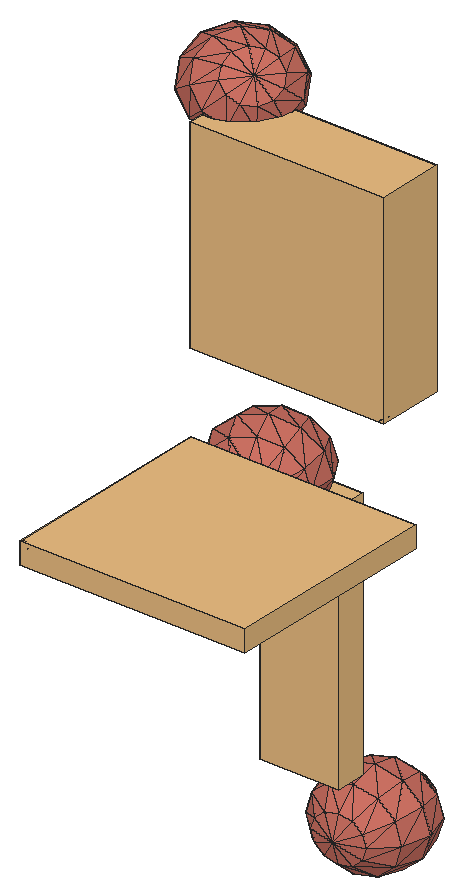
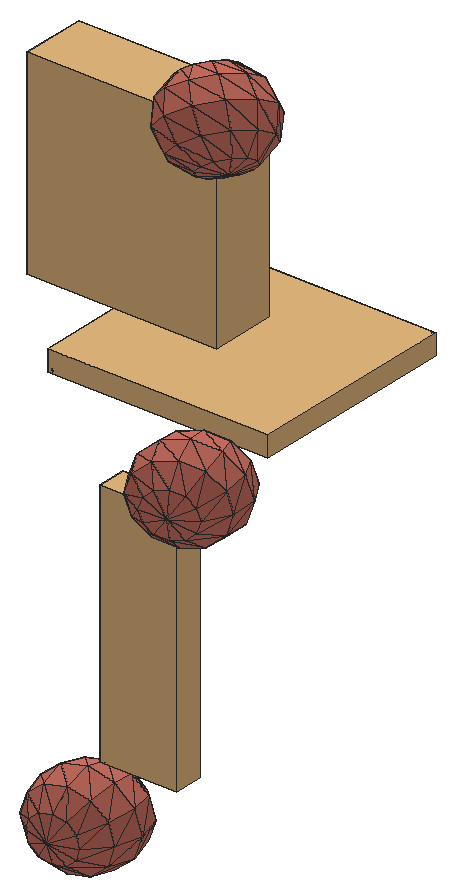
# SketchUp Ruby script. Lengths in inches.
U = 1.inch
M = Sketchup.active_model
def pt(a) = Geom::Point3d.new(a.map { |v| v * U })
def face(e, loops, mat)
  f = e.add_face(loops[0].map { |a| pt(a) })
  loops[1..].each { |l| e.add_face(l.map { |a| pt(a) }).erase! }
  f.material = f.back_material = mat if mat
  f
end
# faces: each face lists its corners as indices into pts; further lists are holes
def faces(e, pts, list, mat = nil) = list.each { |f| face(e, (f[0].is_a?(Array) ? f : [f]).map { |l| l.map { |i| pts[i] } }, mat) }
# xy, xz, yz: faces in a plane at the given z, y or x. An outline is a flat list of corners, or four numbers for a rectangle; further outlines are holes
def ring(l) = l.size == 4 ? [[l[0], l[1]], [l[2], l[1]], [l[2], l[3]], [l[0], l[3]]] : l.each_slice(2).to_a
def flat(e, list, mat, &to3) = list.each { |f| face(e, (f[0].is_a?(Array) ? f : [f]).map { |l| ring(l).map { |u, v| to3.(u, v) } }, mat) }
def xy(e, z, list, mat = nil) = flat(e, list, mat) { |x, y| [x, y, z] }
def xz(e, y, list, mat = nil) = flat(e, list, mat) { |x, z| [x, y, z] }
def yz(e, x, list, mat = nil) = flat(e, list, mat) { |y, z| [x, y, z] }
def lines(e, pts, list) = list.each { |a, b| e.add_line(pt(pts[a]), pt(pts[b])) }
# prism: a flat outline (further loops are holes) pulled along v
def prism(e, loops, v, mat = nil)
  f = face(e, loops, mat); d = Geom::Vector3d.new(v.map { |x| x * U })
  f.pushpull(f.normal.samedirection?(d) ? d.length : -d.length)
end
def box(e, o, s, mat = nil) = prism(e, [[o, [o[0] + s[0], o[1], o[2]], [o[0] + s[0], o[1] + s[1], o[2]], [o[0], o[1] + s[1], o[2]]]], [0, 0, s[2]], mat)
def at(x, y, z, deg = 0) = Geom::Transformation.translation(pt([x, y, z])) * Geom::Transformation.rotation(ORIGIN, Z_AXIS, deg.degrees)
def axes(o, x, y, z) = Geom::Transformation.new([*x, 0, *y, 0, *z, 0, *pt(o).to_a, 1])
def part(name) = M.definitions.add(name)
# library, detail: a bought-in or finely detailed component or shape, given as its bounding box
def library(name, o, s) = part(name).tap { |d| box(d.entities, o, s) }
def detail(e, o, s) = box(e.add_group.entities, o, s)
def put(e, d, t, mat = nil) = e.add_instance(d, t).tap { |i| i.material = mat if mat }
def group(e, t, mat = nil) = e.add_group.tap { |g| g.transformation = t; g.material = mat if mat }.entities
root = M.entities
M.materials.add("green").color = [174, 139, 102]
M.materials.add("vio").color = [206, 114, 100]
c1 = part("3DGeom~243_Defintion")
p = [[-200.91,-81.6,-448.49],[84.65,14.19,-493.26],[-94.16,-142.9,-462.11],[213.68,-130.85,-425.83],[389.77,0,-314.38],[-100.26,120.37,-469.67],
  [240.77,167.48,-392.24],[389.77,0,-314.38],[-311.32,-59.16,-385.97],[-291.49,159.24,-361.38],[27.26,290.09,-365],[-19.66,-226.64,-423.18],
  [-247.73,-261.7,-307.14],[-247.73,-261.7,-307.14],[-247.73,-261.7,-307.14],[252.27,-275.9,-285.45],[213.68,-130.85,-425.83],[434.32,-167.48,-152.28],
  [252.27,-275.9,-285.45],[213.68,-130.85,-425.83],[389.77,0,-314.38],[2.62,-310.38,-342.13],[-247.73,-261.7,-307.14],[252.27,-275.9,-285.45],
  [2.62,-310.38,-342.13],[240.77,167.48,-392.24],[461.41,130.85,-118.6875],[240.77,167.48,-392.24],[332.38,275.9,-186.12],[332.38,275.9,-186.12],
  [-395.79,-81.6,-291.3],[-247.73,-261.7,-307.14],[-395.79,-81.6,-291.3],[-291.49,159.24,-361.38],[-311.32,-59.16,-385.97],[-193.55,334.96,-239.96],
  [147.48,382.07,-162.53],[332.38,275.9,-186.12],[-193.55,334.96,-239.96],[147.48,382.07,-162.53],[27.26,290.09,-365],[-395.79,-81.6,-291.3],
  [-437.8,120.37,-197.41],[-291.49,159.24,-361.38],[-193.55,334.96,-239.96],[-291.49,159.24,-361.38],[2.62,-310.38,-342.13],[190.07,-382.08,-109.73],
  [-33.29,-371.6875,-240.68],[252.27,-275.9,-285.45],[-247.73,-261.7,-307.14],[500,-14.19,21.69],[-117.77,-394.125,-146.01],[-228.17,-371.6875,-83.49],
  [-334.93,-310.38,-69.87],[-334.93,-310.38,-69.87],[-409.43,-226.64,-108.8],[-247.73,-261.7,-307.14],[-431.7,-142.9,-189.85],[-395.79,-81.6,-291.3],
  [-247.73,-261.7,-307.14],[-247.73,-261.7,-307.14],[-395.79,-81.6,-291.3],[252.27,-275.9,-285.45],[362.5,-290.09,50.625],[190.07,-382.08,-109.73],
  [252.27,-275.9,-285.45],[362.5,-290.09,50.625],[43.75,-420.9375,54.25],[-362.5,290.09,-50.625],[-193.55,334.96,-239.96],[-362.5,290.09,-50.625],
  [-43.75,420.9375,-54.25],[-193.55,334.96,-239.96],[-193.55,334.96,-239.96],[147.48,382.07,-162.53],[-500,14.19,-21.69],[409.43,226.64,108.8],
  [334.93,310.39,69.87],[147.48,382.07,-162.53],[334.93,310.39,69.87],[332.38,275.9,-186.12],[147.48,382.07,-162.53],[228.17,371.6875,83.49],
  [334.93,310.39,69.87],[147.48,382.07,-162.53],[437.8,-120.37,197.41],[362.5,-290.09,50.625],[-147.48,-382.08,162.53],[431.7,142.9,189.85],
  [193.55,-334.97,239.96],[362.5,-290.09,50.625],[-461.41,-130.85,118.6875],[-332.38,-275.9,186.12],[-332.38,-275.9,186.12],[-334.93,-310.38,-69.87],
  [-332.38,-275.9,186.12],[-362.5,290.09,-50.625],[-190.07,382.08,109.73],[117.77,394.125,146.01],[-434.32,167.48,152.28],[-190.07,382.08,109.73],
  [395.79,81.6,291.3],[362.5,-290.09,50.625],[291.49,-159.24,361.38],[193.55,-334.97,239.96],[362.5,-290.09,50.625],[-27.26,-290.09,365],
  [-27.26,-290.09,365],[247.73,261.7,307.14],[334.93,310.39,69.87],[247.73,261.7,307.14],[247.73,261.7,307.14],[247.73,261.7,307.14],
  [-252.27,275.9,285.45],[-190.07,382.08,109.73],[-252.27,275.9,285.45],[33.29,371.6875,240.68],[-389.77,0,314.38],[247.73,261.7,307.14],
  [-147.48,-382.08,162.53],[-240.77,-167.48,392.24],[-332.38,-275.9,186.12],[-147.48,-382.08,162.53],[-27.26,-290.09,365],[-240.77,-167.48,392.24],
  [-240.77,-167.48,392.24],[247.73,261.7,307.14],[311.32,59.16,385.97],[193.55,-334.97,239.96],[100.26,-120.37,469.67],[193.55,-334.97,239.96],
  [291.49,-159.24,361.38],[-2.62,310.39,342.13],[247.73,261.7,307.14],[-252.27,275.9,285.45],[-213.68,130.85,425.83],[-213.68,130.85,425.83],
  [-2.62,310.39,342.13],[-252.27,275.9,285.45],[311.32,59.16,385.97],[395.79,81.6,291.3],[247.73,261.7,307.14],[200.91,81.6,448.49],
  [311.32,59.16,385.97],[94.16,142.9,462.11],[19.66,226.64,423.18],[-2.62,310.39,342.13],[-240.77,-167.48,392.24],[-213.68,130.85,425.83],
  [-389.77,0,314.38],[-213.68,130.85,425.83],[-2.62,310.39,342.13],[291.49,-159.24,361.38],[291.49,-159.24,361.38],[311.32,59.16,385.97],
  [-84.65,-14.19,493.26],[-240.77,-167.48,392.24],[-240.77,-167.48,392.24],[-213.68,130.85,425.83],[-213.68,130.85,425.83]]
faces(c1.entities,p,[[0,1,2],[2,1,3],[1,4,3],[0,5,1],[1,6,7],[5,6,1],[8,5,0],[8,9,5],
  [9,10,5],[5,10,6],[2,11,12],[0,2,13],[2,3,11],[8,0,14],[11,3,15],[16,17,18],
  [19,20,17],[11,21,22],[11,23,24],[25,26,20],[27,28,26],[10,29,6],[30,8,31],[32,33,34],
  [9,35,10],[10,36,37],[38,39,40],[41,42,43],[42,44,45],[46,47,48],[46,49,47],[46,48,50],
  [20,51,17],[20,26,51],[48,52,50],[52,53,50],[53,54,50],[55,56,57],[58,59,60],[56,58,61],
  [58,42,62],[63,64,65],[66,17,67],[48,68,52],[48,47,68],[42,69,70],[71,72,73],[74,72,75],
  [58,76,42],[76,69,42],[56,76,58],[28,77,26],[28,78,77],[79,80,81],[82,83,84],[72,83,85],
  [17,86,87],[17,51,86],[52,68,88],[52,88,53],[26,89,51],[26,77,89],[47,90,68],[47,91,90],
  [55,92,56],[56,92,76],[53,88,93],[53,94,95],[55,96,92],[97,98,72],[72,99,83],[98,99,72],
  [76,100,69],[100,101,69],[92,100,76],[51,102,86],[51,89,102],[103,104,105],[106,86,104],[68,107,88],
  [68,90,108],[77,78,109],[110,83,111],[83,99,112],[89,77,113],[100,114,115],[116,117,98],[98,117,99],
  [96,118,92],[92,118,100],[99,117,119],[118,114,100],[120,121,122],[123,124,125],[96,126,118],[102,89,127],
  [86,128,104],[86,102,128],[129,130,124],[131,132,130],[117,133,134],[135,133,117],[118,136,114],[137,138,139],
  [140,141,142],[143,144,142],[145,143,142],[146,145,142],[147,146,142],[148,149,150],[151,146,152],[153,143,130],
  [154,155,143],[124,156,157],[124,130,156],[158,156,159],[156,146,160],[156,145,146],[130,143,145],[130,145,156]],"vio")
c2 = part("3DGeom~210_Defintion")
p = [[-113.26,0,-500],[131.5625,-217.6,-424.04],[-130.88,-188.44,-443.1875],[151.92,0,-489.64],[-348.08,0,-376.38],[-358.26,108.8,-343.58],
  [-130.88,188.44,-443.1875],[-358.26,108.8,-343.58],[-348.08,0,-376.38],[358.76,-188.44,-291.27],[376.38,0,-348.08],[358.76,-188.44,-291.27],
  [131.5625,217.6,-424.04],[75.96,-376.89,-244.82],[-179.04,-326.4,-287.98],[75.96,-376.89,-244.82],[-358.26,-108.8,-343.58],[-179.04,-326.4,-287.98],
  [-348.08,0,-376.38],[-358.26,-108.8,-343.58],[-386.0625,188.44,-253.97],[-358.26,108.8,-343.58],[-386.0625,188.44,-253.97],[-179.04,326.4,-287.98],
  [131.5625,-217.6,-424.04],[310.6,-326.4,-136.0625],[75.96,-376.89,-244.82],[131.5625,-217.6,-424.04],[358.76,-188.44,-291.27],[358.76,188.44,-291.27],
  [75.96,376.89,-244.82],[358.76,188.44,-291.27],[131.5625,217.6,-424.04],[75.96,376.89,-244.82],[-348.08,0,-376.38],[-358.26,-108.8,-343.58],
  [-489.64,0,-151.92],[-358.26,108.8,-343.58],[376.38,0,-348.08],[489.82,-108.8,-80.46],[358.76,-188.44,-291.27],[376.38,0,-348.08],
  [500,0,-113.26],[358.76,188.44,-291.27],[376.38,0,-348.08],[-358.26,-108.8,-343.58],[-179.04,-326.4,-287.98],[-386.0625,-188.44,-253.97],
  [-386.0625,-188.44,-253.97],[-386.0625,188.44,-253.97],[358.76,-188.44,-291.27],[462.02,-188.44,9.15],[310.6,-326.4,-136.0625],[358.76,-188.44,-291.27],
  [358.76,188.44,-291.27],[489.82,108.8,-80.46],[310.6,326.4,-136.0625],[358.76,188.44,-291.27],[75.96,376.89,-244.82],[310.6,326.4,-136.0625],
  [358.76,188.44,-291.27],[-179.04,-326.4,-287.98],[0,-435.19,0],[-244.82,-376.89,-75.96],[-179.04,-326.4,-287.98],[-179.04,-326.4,-287.98],
  [-244.82,-376.89,-75.96],[-424.04,217.6,-131.5625],[-179.04,326.4,-287.98],[-244.82,376.89,-75.96],[-179.04,326.4,-287.98],[-244.82,376.89,-75.96],
  [75.96,376.89,-244.82],[-179.04,326.4,-287.98],[-424.04,-217.6,-131.5625],[244.82,-376.89,75.96],[0,435.19,0],[75.96,376.89,-244.82],
  [-244.82,376.89,-75.96],[75.96,376.89,-244.82],[-462.02,-188.44,-9.15],[-489.82,-108.8,80.46],[-500,0,113.26],[-489.82,108.8,80.46],
  [-462.02,188.44,-9.15],[310.6,-326.4,-136.0625],[424.04,-217.6,131.5625],[244.82,-376.89,75.96],[310.6,-326.4,-136.0625],[310.6,326.4,-136.0625],
  [462.02,188.44,9.15],[244.82,376.89,75.96],[310.6,326.4,-136.0625],[244.82,376.89,75.96],[-310.6,-326.4,136.0625],[489.64,0,151.92],
  [-244.82,-376.89,-75.96],[-75.96,-376.89,244.82],[-244.82,-376.89,-75.96],[-310.6,-326.4,136.0625],[-310.6,326.4,136.0625],[-310.6,326.4,136.0625],
  [-244.82,376.89,-75.96],[-358.76,-188.44,291.27],[179.04,-326.39,287.98],[179.04,-326.39,287.98],[-310.6,326.4,136.0625],[-75.96,376.89,244.82],
  [424.04,217.6,131.5625],[244.82,376.89,75.96],[244.82,-376.89,75.96],[386.0625,-188.44,253.97],[179.04,-326.39,287.98],[244.82,-376.89,75.96],
  [386.0625,-188.44,253.97],[179.04,326.4,287.98],[244.82,376.89,75.96],[179.04,326.4,287.98],[-376.38,0,348.08],[-358.76,188.44,291.27],
  [386.0625,-188.44,253.97],[386.0625,188.44,253.97],[179.04,326.4,287.98],[-310.6,-326.4,136.0625],[-131.5625,-217.6,424.04],[-310.6,-326.4,136.0625],
  [-131.5625,-217.6,424.04],[-358.76,-188.44,291.27],[-358.76,188.44,291.27],[-310.6,326.4,136.0625],[358.26,-108.8,343.58],[386.0625,-188.44,253.97],
  [348.08,0,376.38],[358.26,-108.8,343.58],[358.26,108.8,343.58],[348.08,0,376.38],[358.26,108.8,343.58],[-75.96,-376.89,244.82],
  [130.88,-188.44,443.1875],[-131.5625,-217.6,424.04],[-75.96,-376.89,244.82],[179.04,-326.39,287.98],[-358.76,188.44,291.27],[-131.5625,217.6,424.04],
  [-131.5625,217.6,424.04],[179.04,326.4,287.98],[-75.96,376.89,244.82],[386.0625,-188.44,253.97],[358.26,-108.8,343.58],[130.88,188.44,443.1875],
  [358.26,108.8,343.58],[386.0625,188.44,253.97],[386.0625,188.44,253.97],[179.04,326.4,287.98],[-131.5625,217.6,424.04],[179.04,326.4,287.98],
  [-358.76,-188.44,291.27],[-151.92,0,489.64],[-358.76,-188.44,291.27],[-376.38,0,348.08],[-376.38,0,348.08],[-131.5625,217.6,424.04],
  [-358.76,188.44,291.27],[348.08,0,376.38],[113.26,0,500],[-376.38,0,348.08],[-131.5625,217.6,424.04],[-131.5625,217.6,424.04]]
faces(c2.entities,p,[[0,1,2],[0,3,1],[4,0,2],[5,6,0],[7,0,8],[6,3,0],[3,9,1],[3,10,11],
  [6,12,3],[12,10,3],[2,13,14],[2,1,15],[16,2,17],[18,2,19],[20,6,21],[22,23,6],
  [23,12,6],[24,25,26],[27,28,25],[12,29,10],[30,31,32],[23,33,12],[34,35,36],[37,34,36],
  [38,39,40],[41,42,39],[43,42,44],[45,46,47],[35,48,36],[49,37,36],[50,51,52],[53,39,51],
  [54,55,42],[56,55,57],[58,59,60],[61,62,63],[64,26,62],[48,65,66],[67,68,49],[67,69,70],
  [71,72,73],[48,66,74],[48,74,36],[67,49,36],[26,75,62],[26,25,75],[76,59,77],[78,76,79],
  [74,80,36],[80,81,36],[81,82,36],[82,83,36],[83,84,36],[84,67,36],[85,86,87],[88,51,86],
  [89,90,55],[91,90,92],[76,93,59],[74,66,94],[74,94,80],[84,69,67],[39,42,95],[42,55,95],
  [51,39,95],[55,90,95],[96,62,97],[98,97,99],[84,100,69],[101,76,102],[80,94,103],[80,103,81],
  [83,100,84],[62,104,97],[62,75,105],[106,107,76],[107,93,76],[86,51,95],[90,108,95],[109,108,90],
  [110,111,112],[113,86,114],[115,108,116],[107,117,93],[81,103,118],[81,118,82],[82,119,83],[83,119,100],
  [82,118,119],[120,86,95],[108,121,95],[122,121,108],[123,97,124],[125,126,127],[128,107,129],[130,131,95],
  [132,133,95],[134,135,95],[121,136,95],[137,138,139],[140,141,138],[142,143,107],[144,145,146],[141,147,148],
  [149,150,151],[149,152,153],[141,148,138],[154,149,155],[156,139,157],[158,157,159],[160,161,162],[138,148,163],
  [164,163,150],[164,150,149],[165,157,166],[138,163,164],[139,164,157],[139,138,164],[157,149,167],[157,164,149]],"vio")
c3 = library("3DGeom~78_Defintion",[-59.29,-500,-155.55],[118.58,1000,311.1])
c4 = part("3DGeom~79_Defintion")
p = [[38.96,500,-125.75],[48.07,490.68,-155.1],[39.67,491.3,-155.55],[38.96,500,-125.75],[39.67,491.3,-155.55],[32.3,493.01,-151.95],
  [38.96,500,-125.75],[55.25,491.3,-150.72],[48.07,490.68,-155.1],[38.96,500,-125.75],[32.3,493.01,-151.95],[27.93,495.34,-145.26],
  [38.96,500,-125.75],[59.29,493.01,-143.58],[55.25,491.3,-150.72],[38.96,500,-125.75],[27.93,495.34,-145.26],[27.74,497.67,-137.28],
  [38.96,500,-125.75],[59.1,495.34,-135.59],[59.29,493.01,-143.58],[38.96,500,-125.75],[27.74,497.67,-137.28],[31.78,499.375,-130.14],
  [38.96,500,-125.75],[54.74,497.67,-128.9],[59.1,495.34,-135.59],[38.96,500,-125.75],[47.37,499.375,-125.3],[54.74,497.67,-128.9],
  [-35.57,-494.09,114.48],[-51.43,-495.57,117.9],[-44,-494.49,114.1],[-35.57,-494.09,114.48],[-45.02,-500,144.93],[-51.43,-495.57,117.9],
  [-24.4375,-495.57,126.28],[-45.02,-500,144.93],[-35.57,-494.09,114.48],[-24.4375,-495.57,126.28],[-35.57,-494.09,114.48],[-28.41,-494.49,118.9375],
  [-51.43,-495.57,117.9],[-45.02,-500,144.93],[-56.15,-498.52,133.13],[-51.43,-495.57,117.9],[-56.15,-498.52,133.13],[-55.88,-497.04,124.87],
  [-29.16,-498.52,141.51],[-45.02,-500,144.93],[-24.4375,-495.57,126.28],[-29.16,-498.52,141.51],[-24.4375,-495.57,126.28],[-24.71,-497.04,134.54],
  [-45.02,-500,144.93],[-52.18,-499.6,140.47],[-56.15,-498.52,133.13],[-45.02,-500,144.93],[-29.16,-498.52,141.51],[-36.59,-499.6,145.31]]
faces(c4.entities,p,[[0,1,2],[3,4,5],[6,7,8],[9,10,11],[12,13,14],[15,16,17],[18,19,20],[21,22,23],
  [24,25,26],[27,28,29],[30,31,32],[33,34,35],[36,37,38],[39,40,41],[42,43,44],[45,46,47],
  [48,49,50],[51,52,53],[54,55,56],[57,58,59]],"green")
c5 = part("3DGeom~216_Defintion")
p = [[-234.26,0,-442.1],[18.17,0,-500],[15.74,-212.36,-433.01],[263.63,-183.91,-365.91],[265.74,0,-423.93],[-236.37,183.91,-384.09],
  [15.74,212.36,-433.01],[-236.37,-183.91,-384.09],[-423.93,0,-265.74],[-236.37,-183.91,-384.09],[-425.14,106.18,-232.25],[-425.14,106.18,-232.25],
  [-423.93,0,-265.74],[-236.37,-183.91,-384.09],[9.09,-367.82,-250],[257.87,-318.54,-207.42],[9.09,-367.82,-250],[257.87,-318.54,-207.42],
  [263.63,183.91,-365.91],[-242.13,318.54,-225.59],[9.09,367.82,-250],[-242.13,318.54,-225.59],[265.74,0,-423.93],[440.88,-106.18,-200.77],
  [263.63,-183.91,-365.91],[265.74,0,-423.93],[442.1,0,-234.26],[263.63,183.91,-365.91],[265.74,0,-423.93],[-236.37,-183.91,-384.09],
  [9.09,-367.82,-250],[-242.13,-318.54,-225.59],[-425.14,-106.18,-232.25],[-236.37,-183.91,-384.09],[-242.13,-318.54,-225.59],[-423.93,0,-265.74],
  [-236.37,-183.91,-384.09],[-425.14,-106.18,-232.25],[-428.47,183.91,-140.74],[-236.37,183.91,-384.09],[-425.14,106.18,-232.25],[-242.13,318.54,-225.59],
  [-236.37,183.91,-384.09],[263.63,-183.91,-365.91],[437.56,-183.91,-109.26],[257.87,-318.54,-207.42],[263.63,-183.91,-365.91],[263.63,183.91,-365.91],
  [440.88,106.18,-200.77],[257.87,318.54,-207.42],[263.63,183.91,-365.91],[257.87,318.54,-207.42],[-423.93,0,-265.74],[-500,0,-18.17],
  [-242.13,-318.54,-225.59],[9.09,-367.82,-250],[0,-424.72,0],[250,-367.82,9.09],[257.87,-318.54,-207.42],[-250,367.82,-9.09],
  [9.09,367.82,-250],[-242.13,318.54,-225.59],[0,424.72,0],[257.87,318.54,-207.42],[9.09,367.82,-250],[-250,367.82,-9.09],
  [9.09,367.82,-250],[500,0,18.17],[-428.47,-183.91,-140.74],[-242.13,-318.54,-225.59],[-250,-367.82,-9.09],[-250,-367.82,-9.09],
  [-433.01,212.36,-15.74],[-250,367.82,-9.09],[257.87,-318.54,-207.42],[433.01,-212.36,15.74],[250,-367.82,9.09],[257.87,-318.54,-207.42],
  [257.87,318.54,-207.42],[437.56,183.91,-109.26],[250,367.82,9.09],[257.87,318.54,-207.42],[250,367.82,9.09],[257.87,318.54,-207.42],
  [-433.01,-212.36,-15.74],[433.01,212.36,15.74],[250,367.82,9.09],[-437.56,-183.91,109.26],[-440.88,-106.18,200.77],[-442.1,0,234.26],
  [-437.56,183.91,109.26],[-440.88,106.18,200.77],[-257.87,-318.54,207.42],[-250,-367.82,-9.09],[-9.09,-367.82,250],[-250,-367.82,-9.09],
  [-9.09,-367.82,250],[-257.87,-318.54,207.42],[-257.87,318.54,207.42],[-257.87,318.54,207.42],[-250,367.82,-9.09],[242.13,-318.54,225.59],
  [-9.09,-367.82,250],[242.13,-318.54,225.59],[-257.87,318.54,207.42],[-9.09,367.82,250],[250,-367.82,9.09],[428.47,-183.91,140.74],
  [242.13,-318.54,225.59],[250,-367.82,9.09],[242.13,318.54,225.59],[250,367.82,9.09],[242.13,318.54,225.59],[428.47,183.91,140.74],
  [242.13,318.54,225.59],[425.14,-106.18,232.25],[423.93,0,265.74],[425.14,-106.18,232.25],[425.14,106.18,232.25],[423.93,0,265.74],
  [-263.63,-183.91,365.91],[242.13,-318.54,225.59],[425.14,-106.18,232.25],[236.37,183.91,384.09],[236.37,183.91,384.09],[242.13,318.54,225.59],
  [-265.74,0,423.93],[-263.63,183.91,365.91],[-257.87,-318.54,207.42],[-9.09,-367.82,250],[-15.74,-212.36,433.01],[-257.87,-318.54,207.42],
  [-263.63,-183.91,365.91],[-263.63,183.91,365.91],[-9.09,367.82,250],[-257.87,318.54,207.42],[242.13,-318.54,225.59],[236.37,-183.91,384.09],
  [242.13,-318.54,225.59],[425.14,-106.18,232.25],[236.37,-183.91,384.09],[-15.74,212.36,433.01],[236.37,183.91,384.09],[242.13,318.54,225.59],
  [-9.09,367.82,250],[425.14,-106.18,232.25],[423.93,0,265.74],[234.26,0,442.1],[425.14,106.18,232.25],[425.14,106.18,232.25],
  [-263.63,183.91,365.91],[-9.09,367.82,250],[-263.63,-183.91,365.91],[-18.17,0,500],[-263.63,-183.91,365.91],[-265.74,0,423.93],
  [-265.74,0,423.93],[-263.63,183.91,365.91],[-265.74,0,423.93]]
faces(c5.entities,p,[[0,1,2],[1,3,2],[1,4,3],[5,6,1],[5,1,0],[6,4,1],[0,2,7],[8,0,9],
  [10,5,0],[11,0,12],[13,2,14],[2,15,16],[2,3,17],[6,18,4],[19,6,5],[20,18,6],
  [21,20,6],[22,23,24],[25,26,23],[27,26,28],[29,30,31],[32,33,34],[35,36,37],[38,39,40],
  [38,41,42],[43,44,45],[46,23,44],[47,48,26],[49,48,50],[20,51,18],[52,32,53],[40,52,53],
  [54,55,56],[55,57,56],[55,58,57],[59,60,61],[62,63,64],[65,62,66],[23,26,67],[26,48,67],
  [32,34,68],[32,68,53],[38,40,53],[69,56,70],[68,34,71],[72,41,38],[72,73,41],[74,75,76],
  [77,44,75],[78,79,48],[80,79,81],[62,82,83],[44,23,67],[48,79,67],[68,71,84],[68,84,53],
  [72,38,53],[75,44,67],[79,85,67],[86,85,79],[84,87,53],[87,88,53],[88,89,53],[90,72,53],
  [91,90,53],[89,91,53],[84,71,92],[84,92,87],[90,73,72],[93,56,94],[95,96,97],[90,98,73],
  [99,62,100],[56,101,102],[56,57,103],[104,105,62],[105,82,62],[106,107,108],[109,75,107],[110,85,111],
  [105,112,82],[107,75,67],[85,113,67],[114,113,85],[115,107,67],[116,117,67],[118,119,67],[113,118,67],
  [87,92,120],[87,120,88],[91,98,90],[121,107,122],[123,118,113],[124,113,125],[88,120,126],[88,126,89],
  [89,127,91],[91,127,98],[128,129,130],[131,130,132],[133,134,135],[129,136,137],[138,139,140],[141,142,143],
  [141,143,144],[137,145,146],[147,146,148],[147,149,142],[89,126,127],[129,137,130],[150,141,151],[137,146,147],
  [152,130,153],[154,153,155],[156,141,157],[130,137,147],[153,147,142],[153,142,141],[158,153,141],[130,147,153]],"vio")
c6 = library("3DGeom~171_Defintion",[-163.52,-500,-478.3],[327.04,1000,956.6])
c7 = part("3DGeom~172_Defintion")
p = [[-160.83,493.0625,-454.31],[-133.02,479.16,-476.94],[-143.16,476.9375,-478.3],[-160.83,493.0625,-454.31],[-153.32,477.81,-475.6],[-160.83,493.0625,-454.31],
  [-125.62,483.875,-471.85],[-160.83,493.0625,-454.31],[-153.32,477.81,-475.6],[-160.77,481.53,-469.53],[-160.83,493.0625,-454.31],[-122.93,489.82,-464.42],
  [-125.62,483.875,-471.85],[-160.83,493.0625,-454.31],[-160.77,481.53,-469.53],[-163.52,487.11,-461.74],[-160.83,493.0625,-454.31],[-125.68,495.41,-456.63],
  [-122.93,489.82,-464.42],[-160.83,493.0625,-454.31],[-133.13,499.13,-450.57],[-125.68,495.41,-456.63],[-160.83,493.0625,-454.31],[-153.43,497.78,-449.23],
  [-143.29,500,-447.86],[-160.83,493.0625,-454.31],[-143.29,500,-447.86],[-133.13,499.13,-450.57],[160.33,-486.4,444.8],[144.67,-497.09,441.27],
  [153.43,-492.12,440.5],[144.67,-497.09,441.27],[132.66,-492.22,474],[130.84,-500,455.87],[144.67,-497.09,441.27],[130.84,-500,455.87],
  [136.4,-499.97,446.89],[160.33,-486.4,444.8],[132.66,-492.22,474],[144.67,-497.09,441.27],[162.15,-478.62,462.94],[132.66,-492.22,474],
  [160.33,-486.4,444.8],[162.15,-478.62,462.94],[160.33,-486.4,444.8],[163.52,-481.46,453.02],[132.66,-492.22,474],[129.47,-497.16,465.79],
  [130.84,-500,455.87],[148.32,-481.53,477.54],[132.66,-492.22,474],[162.15,-478.62,462.94],[148.32,-481.53,477.54],[162.15,-478.62,462.94],
  [156.59,-478.65,471.92],[132.66,-492.22,474],[148.32,-481.53,477.54],[139.5625,-486.5,478.3]]
faces(c7.entities,p,[[0,1,2],[3,2,4],[5,6,1],[7,8,9],[10,11,12],[13,14,15],[16,17,18],[19,20,21],
  [22,23,24],[25,26,27],[28,29,30],[31,32,33],[34,35,36],[37,38,39],[40,41,42],[43,44,45],
  [46,47,48],[49,50,51],[52,53,54],[55,56,57]],"green")
c8 = library("3DGeom~185_Defintion",[-474.17,-47.42,-500],[948.34,94.84,1000])
c9 = part("3DGeom~186_Defintion")
p = [[474.17,30.45,-478.03],[446.82,25.72,-499.58],[445.25,33.625,-500],[474.17,30.45,-478.03],[445.25,33.625,-500],[447.56,41.1,-497.47],
  [474.17,30.45,-478.03],[451.84,19.51,-496.34],[446.82,25.72,-499.58],[474.17,30.45,-478.03],[447.56,41.1,-497.47],[453.12,46.15,-492.68],
  [474.17,30.45,-478.03],[458.97,16.66,-491.125],[451.84,19.51,-496.34],[474.17,30.45,-478.03],[453.12,46.15,-492.68],[460.45,47.42,-486.91],
  [474.17,30.45,-478.03],[466.3,17.93,-485.35],[458.97,16.66,-491.125],[474.17,30.45,-478.03],[460.45,47.42,-486.91],[467.58,44.57,-481.7],
  [474.17,30.45,-478.03],[471.87,22.98,-480.56],[466.3,17.93,-485.35],[474.17,30.45,-478.03],[467.58,44.57,-481.7],[472.6,38.36,-478.45],
  [-471.62,-44.41,472.73],[-461.42,-33.9375,500],[-474.17,-30.14,466.08],[-471.62,-44.41,472.73],[-474.17,-30.14,466.08],[-473.6875,-38.09,467.3],
  [-474.17,-30.14,466.08],[-461.42,-33.9375,500],[-470.35,-17.77,476.39],[-474.17,-30.14,466.08],[-470.35,-17.77,476.39],[-472.95,-22.71,469.41],
  [-465.24,-46.31,489.69],[-471.62,-44.41,472.73],[-468.53,-47.42,480.93],[-465.24,-46.31,489.69],[-461.42,-33.9375,500],[-471.62,-44.41,472.73],
  [-470.35,-17.77,476.39],[-461.42,-33.9375,500],[-463.97,-19.67,493.35],[-470.35,-17.77,476.39],[-463.97,-19.67,493.35],[-467.06,-16.66,485.15],
  [-461.42,-33.9375,500],[-465.24,-46.31,489.69],[-462.64,-41.37,496.67],[-461.42,-33.9375,500],[-461.9,-25.99,498.78],[-463.97,-19.67,493.35]]
faces(c9.entities,p,[[0,1,2],[3,4,5],[6,7,8],[9,10,11],[12,13,14],[15,16,17],[18,19,20],[21,22,23],
  [24,25,26],[27,28,29],[30,31,32],[33,34,35],[36,37,38],[39,40,41],[42,43,44],[45,46,47],
  [48,49,50],[51,52,53],[54,55,56],[57,58,59]],"green")
g1 = group(root,at(15.3125,38.42,26.21))
put(g1,c1,axes([-1.65,-0.14,9.04],[0,0.00039,0],[0,0,-0.00039],[-0.00039,0,0]),"vio")
g2 = group(root,at(15.3125,38.42,26.21))
put(g2,c2,axes([-1.58,-0.11,7.8125],[0,0.00038,0],[0,0,-0.00038],[-0.00038,0,0]),"vio")
g3 = group(root,at(15.3125,38.42,26.21))
put(g3,c3,axes([-1.46,-0.07,7.32],[0,0.00091,0],[0,0,-0.00091],[-0.00091,0,0]),"green")
put(g3,c4,axes([-1.46,-0.07,7.32],[0,0.00091,0],[0,0,-0.00091],[-0.00091,0,0]),"green")
g4 = group(root,at(15.3125,38.42,26.21))
put(g4,c5,axes([-1.32,0.04,6.71],[0,0.00039,0],[0,0,-0.00039],[-0.00039,0,0]),"vio")
g5 = group(root,at(15.3125,38.42,26.21))
put(g5,c6,axes([-1.3,-0.26,8.65],[0,0.00073,0],[0,0,-0.00073],[-0.00073,0,0]),"green")
put(g5,c7,axes([-1.3,-0.26,8.65],[0,0.00073,0],[0,0,-0.00073],[-0.00073,0,0]),"green")
g6 = group(root,at(15.3125,38.42,26.21))
put(g6,c8,axes([-1.3,-0.69,7.91],[0,0.00081,0],[0,0,-0.00081],[-0.00081,0,0]),"green")
put(g6,c9,axes([-1.3,-0.69,7.91],[0,0.00081,0],[0,0,-0.00081],[-0.00081,0,0]),"green")
